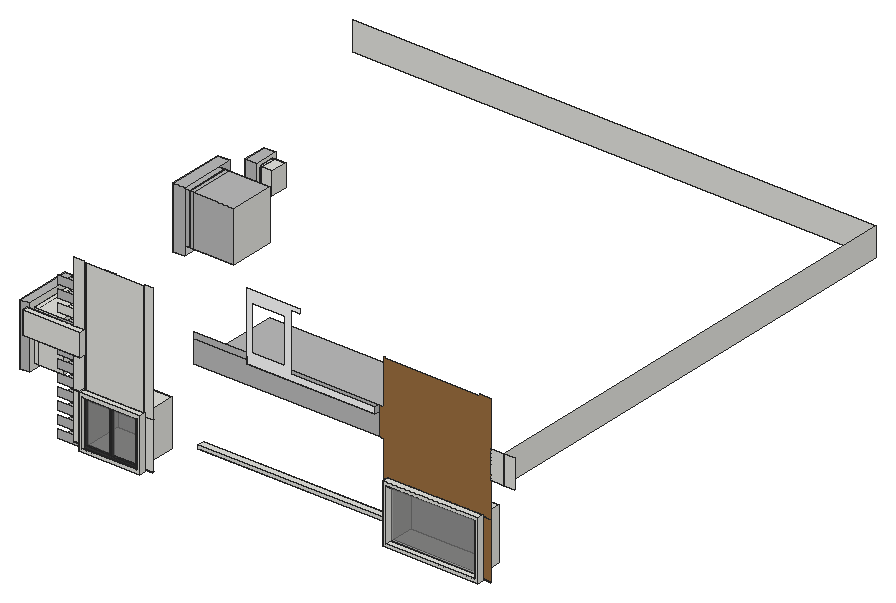
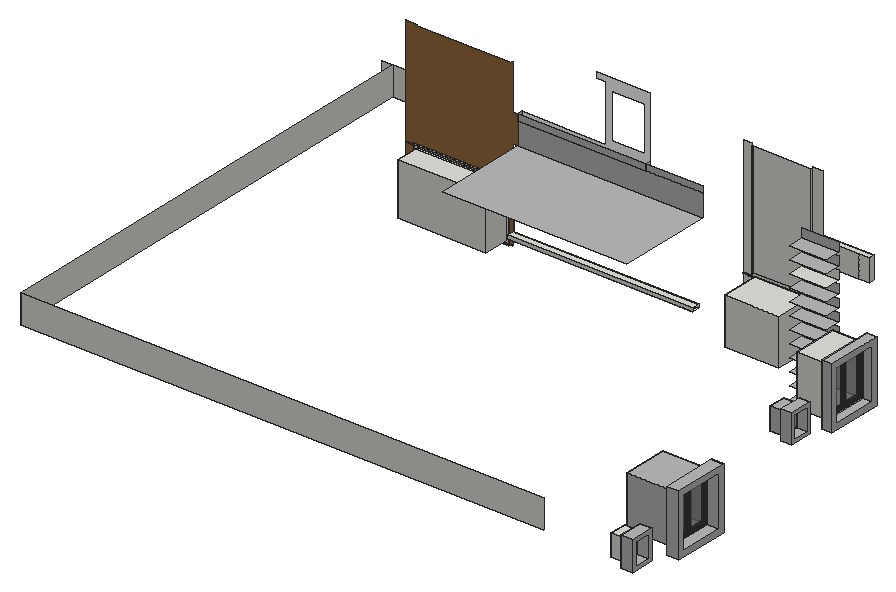
# SketchUp Ruby script. Lengths in inches.
U = 1.inch
M = Sketchup.active_model
def pt(a) = Geom::Point3d.new(a.map { |v| v * U })
def face(e, loops, mat)
  f = e.add_face(loops[0].map { |a| pt(a) })
  loops[1..].each { |l| e.add_face(l.map { |a| pt(a) }).erase! }
  f.material = f.back_material = mat if mat
  f
end
# faces: each face lists its corners as indices into pts; further lists are holes
def faces(e, pts, list, mat = nil) = list.each { |f| face(e, (f[0].is_a?(Array) ? f : [f]).map { |l| l.map { |i| pts[i] } }, mat) }
# xy, xz, yz: faces in a plane at the given z, y or x. An outline is a flat list of corners, or four numbers for a rectangle; further outlines are holes
def ring(l) = l.size == 4 ? [[l[0], l[1]], [l[2], l[1]], [l[2], l[3]], [l[0], l[3]]] : l.each_slice(2).to_a
def flat(e, list, mat, &to3) = list.each { |f| face(e, (f[0].is_a?(Array) ? f : [f]).map { |l| ring(l).map { |u, v| to3.(u, v) } }, mat) }
def xy(e, z, list, mat = nil) = flat(e, list, mat) { |x, y| [x, y, z] }
def xz(e, y, list, mat = nil) = flat(e, list, mat) { |x, z| [x, y, z] }
def yz(e, x, list, mat = nil) = flat(e, list, mat) { |y, z| [x, y, z] }
def lines(e, pts, list) = list.each { |a, b| e.add_line(pt(pts[a]), pt(pts[b])) }
# prism: a flat outline (further loops are holes) pulled along v
def prism(e, loops, v, mat = nil)
  f = face(e, loops, mat); d = Geom::Vector3d.new(v.map { |x| x * U })
  f.pushpull(f.normal.samedirection?(d) ? d.length : -d.length)
end
def box(e, o, s, mat = nil) = prism(e, [[o, [o[0] + s[0], o[1], o[2]], [o[0] + s[0], o[1] + s[1], o[2]], [o[0], o[1] + s[1], o[2]]]], [0, 0, s[2]], mat)
def at(x, y, z, deg = 0) = Geom::Transformation.translation(pt([x, y, z])) * Geom::Transformation.rotation(ORIGIN, Z_AXIS, deg.degrees)
def axes(o, x, y, z) = Geom::Transformation.new([*x, 0, *y, 0, *z, 0, *pt(o).to_a, 1])
def part(name) = M.definitions.add(name)
# library, detail: a bought-in or finely detailed component or shape, given as its bounding box
def library(name, o, s) = part(name).tap { |d| box(d.entities, o, s) }
def detail(e, o, s) = box(e.add_group.entities, o, s)
def put(e, d, t, mat = nil) = e.add_instance(d, t).tap { |i| i.material = mat if mat }
def group(e, t, mat = nil) = e.add_group.tap { |g| g.transformation = t; g.material = mat if mat }.entities
root = M.entities
M.materials.add("Generic").color = [155, 110, 63]
M.materials.add("Generic\#2").color = [186, 186, 186]
M.materials.add("[Color M00]").color = [255, 255, 255]
M.materials.add("[Color M07]").color = [58, 58, 58]
M.materials.add("[Translucent Glass Gray]").color = [127, 127, 127]
M.materials["[Translucent Glass Gray]"].alpha = 0.58
M.materials.add("[Translucent Glass Gray]1").color = [127, 127, 127]
M.materials["[Translucent Glass Gray]1"].alpha = 0.5
c1 = part("Group\#1")
xy(c1.entities,0,[[0,0,46.77,20.375]])
xz(c1.entities,0,[[0,0,46.77,11.0625]])
c2 = part("Group\#3")
xy(c2.entities,0,[[0,0,70.4375,6]],"[Color M07]")
xy(c2.entities,2.83,[[2.83,0,33.8,3],[36.63,0,67.61,3]],"[Color M07]")
xy(c2.entities,56.73,[[2.83,0,33.8,3],[36.63,0,67.61,3]],"[Color M07]")
xy(c2.entities,59.5625,[[0,0,70.4375,6]],"[Color M07]")
xz(c2.entities,0,[[[0,0,70.4375,59.5625],[2.83,2.83,33.8,56.73],[36.63,2.83,67.61,56.73]]],"[Color M07]")
xz(c2.entities,3,[[2.83,2.83,33.8,56.73],[36.63,2.83,67.61,56.73]],"[Translucent Glass Gray]")
xz(c2.entities,6,[[0,0,70.4375,59.5625]],"[Translucent Glass Gray]")
yz(c2.entities,0,[[0,0,6,59.5625]],"[Color M07]")
yz(c2.entities,2.83,[[0,2.83,3,56.73]],"[Color M07]")
yz(c2.entities,33.8,[[0,2.83,3,56.73]],"[Color M07]")
yz(c2.entities,36.63,[[0,2.83,3,56.73]],"[Color M07]")
yz(c2.entities,67.61,[[0,2.83,3,56.73]],"[Color M07]")
yz(c2.entities,70.4375,[[0,0,6,59.5625]],"[Color M07]")
c3 = part("Group\#2")
xy(c3.entities,0,[[0,0,113.875,3]])
xy(c3.entities,67.5625,[[0,0,113.875,3]])
xz(c3.entities,0,[[0,0,113.875,67.5625]],"[Translucent Glass Gray]")
xz(c3.entities,3,[[0,0,113.875,67.5625]],"[Translucent Glass Gray]")
yz(c3.entities,0,[[0,0,3,67.5625]])
yz(c3.entities,113.875,[[0,0,3,67.5625]])
c4 = part("Group\#4")
xy(c4.entities,0,[[0,0,6,57.4375]],"[Color M07]")
xy(c4.entities,5.48,[[0,5.48,3,25.98],[0,31.46,3,51.96]],"[Color M07]")
xy(c4.entities,59.46,[[0,5.48,3,25.98],[0,31.46,3,51.96]],"[Color M07]")
xy(c4.entities,64.9375,[[0,0,6,57.4375]],"[Color M07]")
xz(c4.entities,0,[[0,0,6,64.9375]],"[Color M07]")
xz(c4.entities,5.48,[[0,5.48,3,59.46]],"[Color M07]")
xz(c4.entities,25.98,[[0,5.48,3,59.46]],"[Color M07]")
xz(c4.entities,31.46,[[0,5.48,3,59.46]],"[Color M07]")
xz(c4.entities,51.96,[[0,5.48,3,59.46]],"[Color M07]")
xz(c4.entities,57.4375,[[0,0,6,64.9375]],"[Color M07]")
yz(c4.entities,0,[[[0,0,57.4375,64.9375],[31.46,5.48,51.96,59.46],[5.48,5.48,25.98,59.46]]],"[Color M07]")
yz(c4.entities,3,[[5.48,5.48,25.98,59.46],[31.46,5.48,51.96,59.46]],"[Translucent Glass Gray]1")
yz(c4.entities,6,[[0,0,57.4375,64.9375]],"[Translucent Glass Gray]1")
c5 = part("Group\#5")
xy(c5.entities,0,[[0,0,3,21.5625]])
xy(c5.entities,28.3125,[[0,0,3,21.5625]])
xz(c5.entities,0,[[0,0,3,28.3125]])
xz(c5.entities,21.5625,[[0,0,3,28.3125]])
yz(c5.entities,0,[[0,0,21.5625,28.3125]],"[Translucent Glass Gray]1")
yz(c5.entities,3,[[0,0,21.5625,28.3125]],"[Translucent Glass Gray]1")
xy(root,450.375,[[170.35,89.25,249.19,97.25],[171.66,97.25,172.16,98.375],[247.01,97.25,247.51,98.375]])
xy(root,453.4375,[[157.47,97.25,170.35,98.375],[249.19,97.25,259.3125,98.375]])
xy(root,453.9375,[[157.47,97.25,170.35,98.375],[249.19,97.25,259.3125,98.375]])
xy(root,454.58,[[174.55,89.25,244.99,97.25],[174.55,97.25,244.99,145.8125]])
xy(root,458.4,[[540.25,116.625,662.53,124.5]])
xy(root,461.15,[[0,454.08,15.3125,525.8]],"Generic\#2")
xy(root,462.6,[[544.45,116.625,658.33,124.5],[544.45,124.5,658.33,156.8125]])
xy(root,467.02,[[36.4375,161.95,48.5,234.18]],"Generic\#2")
xy(root,468.29,[[0,461.22,72.5625,518.66]],"Generic\#2")
xy(root,474.41,[[48.5,169.34,87,226.78]])
xy(root,474.41,[[36.4375,169.34,48.5,226.78]],"Generic\#2")
xy(root,477.08,[[[290.4375,131.37,528.75,140.67],[521.23,133.41,521.44,133.44,521.64,133.52,521.8,133.65,521.93,133.82,522.02,134.02,522.04,134.23,522.02,134.4375,521.93,134.63,521.8,134.8,521.64,134.93,521.44,135.01,521.23,135.04,521.02,135.01,520.82,134.93,520.66,134.8,520.53,134.63,520.45,134.4375,520.42,134.23,520.45,134.02,520.53,133.82,520.66,133.65,520.82,133.52,521.02,133.44],[515.92,133.41,516.13,133.44,516.32,133.52,516.49,133.65,516.62,133.82,516.7,134.02,516.73,134.23,516.7,134.4375,516.62,134.63,516.49,134.8,516.32,134.93,516.13,135.01,515.92,135.04,515.71,135.01,515.51,134.93,515.34,134.8,515.21,134.63,515.13,134.4375,515.11,134.23,515.13,134.02,515.21,133.82,515.34,133.65,515.51,133.52,515.71,133.44],[510.67,133.41,510.88,133.44,511.07,133.52,511.24,133.65,511.37,133.82,511.45,134.02,511.48,134.23,511.45,134.4375,511.37,134.63,511.24,134.8,511.07,134.93,510.88,135.01,510.67,135.04,510.46,135.01,510.26,134.93,510.09,134.8,509.96,134.63,509.88,134.4375,509.86,134.23,509.88,134.02,509.96,133.82,510.09,133.65,510.26,133.52,510.46,133.44],[505.42,133.41,505.63,133.44,505.82,133.52,505.99,133.65,506.12,133.82,506.2,134.02,506.23,134.23,506.2,134.4375,506.12,134.63,505.99,134.8,505.82,134.93,505.63,135.01,505.42,135.04,505.21,135.01,505.01,134.93,504.84,134.8,504.71,134.63,504.63,134.4375,504.61,134.23,504.63,134.02,504.71,133.82,504.84,133.65,505.01,133.52,505.21,133.44],[500.17,133.41,500.38,133.44,500.57,133.52,500.74,133.65,500.87,133.82,500.95,134.02,500.98,134.23,500.95,134.4375,500.87,134.63,500.74,134.8,500.57,134.93,500.38,135.01,500.17,135.04,499.96,135.01,499.76,134.93,499.59,134.8,499.46,134.63,499.38,134.4375,499.36,134.23,499.38,134.02,499.46,133.82,499.59,133.65,499.76,133.52,499.96,133.44],[494.86,133.41,495.07,133.44,495.26,133.52,495.43,133.65,495.56,133.82,495.64,134.02,495.67,134.23,495.64,134.4375,495.56,134.63,495.43,134.8,495.26,134.93,495.07,135.01,494.86,135.04,494.65,135.01,494.45,134.93,494.28,134.8,494.15,134.63,494.07,134.4375,494.04,134.23,494.07,134.02,494.15,133.82,494.28,133.65,494.45,133.52,494.65,133.44],[489.54,133.41,489.75,133.44,489.95,133.52,490.12,133.65,490.25,133.82,490.33,134.02,490.36,134.23,490.33,134.4375,490.25,134.63,490.12,134.8,489.95,134.93,489.75,135.01,489.54,135.04,489.33,135.01,489.14,134.93,488.97,134.8,488.84,134.63,488.76,134.4375,488.73,134.23,488.76,134.02,488.84,133.82,488.97,133.65,489.14,133.52,489.33,133.44],[483.92,133.41,484.13,133.44,484.32,133.52,484.49,133.65,484.62,133.82,484.7,134.02,484.73,134.23,484.7,134.4375,484.62,134.63,484.49,134.8,484.32,134.93,484.13,135.01,483.92,135.04,483.71,135.01,483.51,134.93,483.34,134.8,483.21,134.63,483.13,134.4375,483.11,134.23,483.13,134.02,483.21,133.82,483.34,133.65,483.51,133.52,483.71,133.44],[478.67,133.41,478.88,133.44,479.07,133.52,479.24,133.65,479.37,133.82,479.45,134.02,479.48,134.23,479.45,134.4375,479.37,134.63,479.24,134.8,479.07,134.93,478.88,135.01,478.67,135.04,478.46,135.01,478.26,134.93,478.09,134.8,477.96,134.63,477.88,134.4375,477.86,134.23,477.88,134.02,477.96,133.82,478.09,133.65,478.26,133.52,478.46,133.44],[473.42,133.41,473.63,133.44,473.82,133.52,473.99,133.65,474.12,133.82,474.2,134.02,474.23,134.23,474.2,134.4375,474.12,134.63,473.99,134.8,473.82,134.93,473.63,135.01,473.42,135.04,473.21,135.01,473.01,134.93,472.84,134.8,472.71,134.63,472.63,134.4375,472.61,134.23,472.63,134.02,472.71,133.82,472.84,133.65,473.01,133.52,473.21,133.44],[468.17,133.41,468.38,133.44,468.57,133.52,468.74,133.65,468.87,133.82,468.95,134.02,468.98,134.23,468.95,134.4375,468.87,134.63,468.74,134.8,468.57,134.93,468.38,135.01,468.17,135.04,467.96,135.01,467.76,134.93,467.59,134.8,467.46,134.63,467.38,134.4375,467.36,134.23,467.38,134.02,467.46,133.82,467.59,133.65,467.76,133.52,467.96,133.44],[462.92,133.41,463.13,133.44,463.32,133.52,463.49,133.65,463.62,133.82,463.7,134.02,463.73,134.23,463.7,134.4375,463.62,134.63,463.49,134.8,463.32,134.93,463.13,135.01,462.92,135.04,462.71,135.01,462.51,134.93,462.34,134.8,462.21,134.63,462.13,134.4375,462.11,134.23,462.13,134.02,462.21,133.82,462.34,133.65,462.51,133.52,462.71,133.44],[457.67,133.41,457.88,133.44,458.07,133.52,458.24,133.65,458.37,133.82,458.45,134.02,458.48,134.23,458.45,134.4375,458.37,134.63,458.24,134.8,458.07,134.93,457.88,135.01,457.67,135.04,457.46,135.01,457.26,134.93,457.09,134.8,456.96,134.63,456.88,134.4375,456.86,134.23,456.88,134.02,456.96,133.82,457.09,133.65,457.26,133.52,457.46,133.44],[452.36,133.41,452.57,133.44,452.76,133.52,452.93,133.65,453.06,133.82,453.14,134.02,453.17,134.23,453.14,134.4375,453.06,134.63,452.93,134.8,452.76,134.93,452.57,135.01,452.36,135.04,452.15,135.01,451.95,134.93,451.78,134.8,451.65,134.63,451.57,134.4375,451.54,134.23,451.57,134.02,451.65,133.82,451.78,133.65,451.95,133.52,452.15,133.44],[447.04,133.41,447.25,133.44,447.45,133.52,447.62,133.65,447.75,133.82,447.83,134.02,447.86,134.23,447.83,134.4375,447.75,134.63,447.62,134.8,447.45,134.93,447.25,135.01,447.04,135.04,446.83,135.01,446.64,134.93,446.47,134.8,446.34,134.63,446.26,134.4375,446.23,134.23,446.26,134.02,446.34,133.82,446.47,133.65,446.64,133.52,446.83,133.44],[441.73,133.41,441.94,133.44,442.14,133.52,442.3,133.65,442.43,133.82,442.52,134.02,442.54,134.23,442.52,134.4375,442.43,134.63,442.3,134.8,442.14,134.93,441.94,135.01,441.73,135.04,441.52,135.01,441.32,134.93,441.16,134.8,441.03,134.63,440.95,134.4375,440.92,134.23,440.95,134.02,441.03,133.82,441.16,133.65,441.32,133.52,441.52,133.44],[436.42,133.41,436.63,133.44,436.82,133.52,436.99,133.65,437.12,133.82,437.2,134.02,437.23,134.23,437.2,134.4375,437.12,134.63,436.99,134.8,436.82,134.93,436.63,135.01,436.42,135.04,436.21,135.01,436.01,134.93,435.84,134.8,435.71,134.63,435.63,134.4375,435.61,134.23,435.63,134.02,435.71,133.82,435.84,133.65,436.01,133.52,436.21,133.44],[431.11,133.41,431.32,133.44,431.51,133.52,431.68,133.65,431.81,133.82,431.89,134.02,431.92,134.23,431.89,134.4375,431.81,134.63,431.68,134.8,431.51,134.93,431.32,135.01,431.11,135.04,430.9,135.01,430.7,134.93,430.53,134.8,430.4,134.63,430.32,134.4375,430.29,134.23,430.32,134.02,430.4,133.82,430.53,133.65,430.7,133.52,430.9,133.44],[425.79,133.41,426,133.44,426.2,133.52,426.37,133.65,426.5,133.82,426.58,134.02,426.61,134.23,426.58,134.4375,426.5,134.63,426.37,134.8,426.2,134.93,426,135.01,425.79,135.04,425.58,135.01,425.39,134.93,425.22,134.8,425.09,134.63,425.01,134.4375,424.98,134.23,425.01,134.02,425.09,133.82,425.22,133.65,425.39,133.52,425.58,133.44],[420.48,133.41,420.69,133.44,420.89,133.52,421.05,133.65,421.18,133.82,421.27,134.02,421.29,134.23,421.27,134.4375,421.18,134.63,421.05,134.8,420.89,134.93,420.69,135.01,420.48,135.04,420.27,135.01,420.07,134.93,419.91,134.8,419.78,134.63,419.7,134.4375,419.67,134.23,419.7,134.02,419.78,133.82,419.91,133.65,420.07,133.52,420.27,133.44],[415.17,133.41,415.38,133.44,415.57,133.52,415.74,133.65,415.87,133.82,415.95,134.02,415.98,134.23,415.95,134.4375,415.87,134.63,415.74,134.8,415.57,134.93,415.38,135.01,415.17,135.04,414.96,135.01,414.76,134.93,414.59,134.8,414.46,134.63,414.38,134.4375,414.36,134.23,414.38,134.02,414.46,133.82,414.59,133.65,414.76,133.52,414.96,133.44],[409.86,133.41,410.07,133.44,410.26,133.52,410.43,133.65,410.56,133.82,410.64,134.02,410.67,134.23,410.64,134.4375,410.56,134.63,410.43,134.8,410.26,134.93,410.07,135.01,409.86,135.04,409.65,135.01,409.45,134.93,409.28,134.8,409.15,134.63,409.07,134.4375,409.04,134.23,409.07,134.02,409.15,133.82,409.28,133.65,409.45,133.52,409.65,133.44],[404.54,133.41,404.75,133.44,404.95,133.52,405.12,133.65,405.25,133.82,405.33,134.02,405.36,134.23,405.33,134.4375,405.25,134.63,405.12,134.8,404.95,134.93,404.75,135.01,404.54,135.04,404.33,135.01,404.14,134.93,403.97,134.8,403.84,134.63,403.76,134.4375,403.73,134.23,403.76,134.02,403.84,133.82,403.97,133.65,404.14,133.52,404.33,133.44],[399.23,133.41,399.44,133.44,399.64,133.52,399.8,133.65,399.93,133.82,400.02,134.02,400.04,134.23,400.02,134.4375,399.93,134.63,399.8,134.8,399.64,134.93,399.44,135.01,399.23,135.04,399.02,135.01,398.82,134.93,398.66,134.8,398.53,134.63,398.45,134.4375,398.42,134.23,398.45,134.02,398.53,133.82,398.66,133.65,398.82,133.52,399.02,133.44],[393.92,133.41,394.13,133.44,394.32,133.52,394.49,133.65,394.62,133.82,394.7,134.02,394.73,134.23,394.7,134.4375,394.62,134.63,394.49,134.8,394.32,134.93,394.13,135.01,393.92,135.04,393.71,135.01,393.51,134.93,393.34,134.8,393.21,134.63,393.13,134.4375,393.11,134.23,393.13,134.02,393.21,133.82,393.34,133.65,393.51,133.52,393.71,133.44],[388.61,133.41,388.82,133.44,389.01,133.52,389.18,133.65,389.31,133.82,389.39,134.02,389.42,134.23,389.39,134.4375,389.31,134.63,389.18,134.8,389.01,134.93,388.82,135.01,388.61,135.04,388.4,135.01,388.2,134.93,388.03,134.8,387.9,134.63,387.82,134.4375,387.79,134.23,387.82,134.02,387.9,133.82,388.03,133.65,388.2,133.52,388.4,133.44],[383.29,133.41,383.5,133.44,383.7,133.52,383.87,133.65,384,133.82,384.08,134.02,384.11,134.23,384.08,134.4375,384,134.63,383.87,134.8,383.7,134.93,383.5,135.01,383.29,135.04,383.08,135.01,382.89,134.93,382.72,134.8,382.59,134.63,382.51,134.4375,382.48,134.23,382.51,134.02,382.59,133.82,382.72,133.65,382.89,133.52,383.08,133.44],[377.98,133.41,378.19,133.44,378.39,133.52,378.55,133.65,378.68,133.82,378.77,134.02,378.79,134.23,378.77,134.4375,378.68,134.63,378.55,134.8,378.39,134.93,378.19,135.01,377.98,135.04,377.77,135.01,377.57,134.93,377.41,134.8,377.28,134.63,377.2,134.4375,377.17,134.23,377.2,134.02,377.28,133.82,377.41,133.65,377.57,133.52,377.77,133.44],[372.67,133.41,372.88,133.44,373.07,133.52,373.24,133.65,373.37,133.82,373.45,134.02,373.48,134.23,373.45,134.4375,373.37,134.63,373.24,134.8,373.07,134.93,372.88,135.01,372.67,135.04,372.46,135.01,372.26,134.93,372.09,134.8,371.96,134.63,371.88,134.4375,371.86,134.23,371.88,134.02,371.96,133.82,372.09,133.65,372.26,133.52,372.46,133.44],[367.36,133.41,367.57,133.44,367.76,133.52,367.93,133.65,368.06,133.82,368.14,134.02,368.17,134.23,368.14,134.4375,368.06,134.63,367.93,134.8,367.76,134.93,367.57,135.01,367.36,135.04,367.15,135.01,366.95,134.93,366.78,134.8,366.65,134.63,366.57,134.4375,366.54,134.23,366.57,134.02,366.65,133.82,366.78,133.65,366.95,133.52,367.15,133.44],[362.04,133.41,362.25,133.44,362.45,133.52,362.62,133.65,362.75,133.82,362.83,134.02,362.86,134.23,362.83,134.4375,362.75,134.63,362.62,134.8,362.45,134.93,362.25,135.01,362.04,135.04,361.83,135.01,361.64,134.93,361.47,134.8,361.34,134.63,361.26,134.4375,361.23,134.23,361.26,134.02,361.34,133.82,361.47,133.65,361.64,133.52,361.83,133.44],[356.73,133.41,356.94,133.44,357.14,133.52,357.3,133.65,357.43,133.82,357.52,134.02,357.54,134.23,357.52,134.4375,357.43,134.63,357.3,134.8,357.14,134.93,356.94,135.01,356.73,135.04,356.52,135.01,356.32,134.93,356.16,134.8,356.03,134.63,355.95,134.4375,355.92,134.23,355.95,134.02,356.03,133.82,356.16,133.65,356.32,133.52,356.52,133.44],[351.42,133.41,351.63,133.44,351.82,133.52,351.99,133.65,352.12,133.82,352.2,134.02,352.23,134.23,352.2,134.4375,352.12,134.63,351.99,134.8,351.82,134.93,351.63,135.01,351.42,135.04,351.21,135.01,351.01,134.93,350.84,134.8,350.71,134.63,350.63,134.4375,350.61,134.23,350.63,134.02,350.71,133.82,350.84,133.65,351.01,133.52,351.21,133.44],[346.11,133.41,346.32,133.44,346.51,133.52,346.68,133.65,346.81,133.82,346.89,134.02,346.92,134.23,346.89,134.4375,346.81,134.63,346.68,134.8,346.51,134.93,346.32,135.01,346.11,135.04,345.9,135.01,345.7,134.93,345.53,134.8,345.4,134.63,345.32,134.4375,345.29,134.23,345.32,134.02,345.4,133.82,345.53,133.65,345.7,133.52,345.9,133.44],[340.79,133.41,341,133.44,341.2,133.52,341.37,133.65,341.5,133.82,341.58,134.02,341.61,134.23,341.58,134.4375,341.5,134.63,341.37,134.8,341.2,134.93,341,135.01,340.79,135.04,340.58,135.01,340.39,134.93,340.22,134.8,340.09,134.63,340.01,134.4375,339.98,134.23,340.01,134.02,340.09,133.82,340.22,133.65,340.39,133.52,340.58,133.44],[335.48,133.41,335.69,133.44,335.89,133.52,336.05,133.65,336.18,133.82,336.27,134.02,336.29,134.23,336.27,134.4375,336.18,134.63,336.05,134.8,335.89,134.93,335.69,135.01,335.48,135.04,335.27,135.01,335.07,134.93,334.91,134.8,334.78,134.63,334.7,134.4375,334.67,134.23,334.7,134.02,334.78,133.82,334.91,133.65,335.07,133.52,335.27,133.44],[330.17,133.41,330.38,133.44,330.57,133.52,330.74,133.65,330.87,133.82,330.95,134.02,330.98,134.23,330.95,134.4375,330.87,134.63,330.74,134.8,330.57,134.93,330.38,135.01,330.17,135.04,329.96,135.01,329.76,134.93,329.59,134.8,329.46,134.63,329.38,134.4375,329.36,134.23,329.38,134.02,329.46,133.82,329.59,133.65,329.76,133.52,329.96,133.44],[324.86,133.41,325.07,133.44,325.26,133.52,325.43,133.65,325.56,133.82,325.64,134.02,325.67,134.23,325.64,134.4375,325.56,134.63,325.43,134.8,325.26,134.93,325.07,135.01,324.86,135.04,324.65,135.01,324.45,134.93,324.28,134.8,324.15,134.63,324.07,134.4375,324.04,134.23,324.07,134.02,324.15,133.82,324.28,133.65,324.45,133.52,324.65,133.44],[319.54,133.41,319.75,133.44,319.95,133.52,320.12,133.65,320.25,133.82,320.33,134.02,320.36,134.23,320.33,134.4375,320.25,134.63,320.12,134.8,319.95,134.93,319.75,135.01,319.54,135.04,319.33,135.01,319.14,134.93,318.97,134.8,318.84,134.63,318.76,134.4375,318.73,134.23,318.76,134.02,318.84,133.82,318.97,133.65,319.14,133.52,319.33,133.44],[314.23,133.41,314.44,133.44,314.64,133.52,314.8,133.65,314.93,133.82,315.02,134.02,315.04,134.23,315.02,134.4375,314.93,134.63,314.8,134.8,314.64,134.93,314.44,135.01,314.23,135.04,314.02,135.01,313.82,134.93,313.66,134.8,313.53,134.63,313.45,134.4375,313.42,134.23,313.45,134.02,313.53,133.82,313.66,133.65,313.82,133.52,314.02,133.44],[308.92,133.41,309.13,133.44,309.32,133.52,309.49,133.65,309.62,133.82,309.7,134.02,309.73,134.23,309.7,134.4375,309.62,134.63,309.49,134.8,309.32,134.93,309.13,135.01,308.92,135.04,308.71,135.01,308.51,134.93,308.34,134.8,308.21,134.63,308.13,134.4375,308.11,134.23,308.13,134.02,308.21,133.82,308.34,133.65,308.51,133.52,308.71,133.44],[303.61,133.41,303.82,133.44,304.01,133.52,304.18,133.65,304.31,133.82,304.39,134.02,304.42,134.23,304.39,134.4375,304.31,134.63,304.18,134.8,304.01,134.93,303.82,135.01,303.61,135.04,303.4,135.01,303.2,134.93,303.03,134.8,302.9,134.63,302.82,134.4375,302.79,134.23,302.82,134.02,302.9,133.82,303.03,133.65,303.2,133.52,303.4,133.44],[298.29,133.41,298.5,133.44,298.7,133.52,298.87,133.65,299,133.82,299.08,134.02,299.11,134.23,299.08,134.4375,299,134.63,298.87,134.8,298.7,134.93,298.5,135.01,298.29,135.04,298.08,135.01,297.89,134.93,297.72,134.8,297.59,134.63,297.51,134.4375,297.48,134.23,297.51,134.02,297.59,133.82,297.72,133.65,297.89,133.52,298.08,133.44],[292.92,133.41,293.13,133.44,293.32,133.52,293.49,133.65,293.62,133.82,293.7,134.02,293.73,134.23,293.7,134.4375,293.62,134.63,293.49,134.8,293.32,134.93,293.13,135.01,292.92,135.04,292.71,135.01,292.51,134.93,292.34,134.8,292.21,134.63,292.13,134.4375,292.11,134.23,292.13,134.02,292.21,133.82,292.34,133.65,292.51,133.52,292.71,133.44]]])
xy(root,478.92,[[0,569.42,15.3125,600.66]],"Generic\#2")
xy(root,481.27,[[290.4375,131.37,528.75,140.67]])
xy(root,482.8,[[34.5,270.92,48.5,300.91]],"Generic\#2")
xy(root,483.76,[[15.3125,574.26,31.25,595.82]])
xy(root,483.76,[[0,574.26,15.3125,595.82]],"Generic\#2")
xy(root,487.01,[[34.5,275.13,65.625,296.69]],"Generic\#2")
xy(root,512.07,[[15.3125,574.26,31.25,595.82]])
xy(root,512.07,[[0,574.26,15.3125,595.82]],"Generic\#2")
xy(root,513.6875,[[157.47,97.25,170.35,98.375],[249.19,97.25,259.3125,98.375]])
xy(root,514.14,[[174.55,89.25,244.99,97.25],[174.55,97.25,244.99,145.8125]])
xy(root,514.1875,[[157.47,97.25,170.35,98.375],[249.19,97.25,259.3125,98.375]])
xy(root,515.32,[[34.5,275.13,65.625,296.69]],"Generic\#2")
xy(root,516.91,[[0,569.42,15.3125,600.66]],"Generic\#2")
xy(root,518.34,[[170.35,89.25,249.19,97.25],[171.66,97.25,172.16,98.375],[247.01,97.25,247.51,98.375]])
xy(root,519.54,[[34.5,270.92,48.5,300.91]],"Generic\#2")
xy(root,530.16,[[544.45,116.625,658.33,124.5],[544.45,124.5,658.33,156.8125]])
xy(root,533.23,[[0,461.22,72.5625,518.66]],"Generic\#2")
xy(root,534.36,[[540.25,116.625,662.53,124.5]])
xy(root,539.35,[[48.5,169.34,87,226.78]])
xy(root,539.35,[[36.4375,169.34,48.5,226.78]],"Generic\#2")
xy(root,540.37,[[0,454.08,15.3125,525.8]],"Generic\#2")
xy(root,546.75,[[36.4375,161.95,48.5,234.18]],"Generic\#2")
xy(root,558.95,[[96.98,89.5625,171.66,97.25]])
xy(root,577.875,[[290.4375,124.5,528.75,246]],"Generic\#2")
xy(root,587.54,[[96.98,89.5625,171.66,97.25]])
xy(root,606.6875,[[363.4375,118.5625,528.75,124.5]],"Generic\#2")
xz(root,89.25,[[[170.35,450.375,249.19,518.34],[174.55,454.58,244.99,514.14]]])
xz(root,89.5625,[[96.98,558.95,171.66,587.54]])
xz(root,97.25,[[170.35,450.375,171.66,514.1875],[[171.66,450.375,247.01,514.1875],[174.55,454.58,244.99,514.14]],[247.01,450.375,249.19,514.1875],[157.47,453.9375,170.35,513.6875],[249.19,453.9375,259.3125,513.6875],
  [157.47,514.1875,170.35,514.1875,170.35,518.34,171.66,518.34,171.66,558.95,157.47,558.95],[170.35,514.1875,171.66,518.34],[171.66,514.1875,247.01,518.34],[247.01,514.1875,249.19,518.34],[249.19,514.1875,259.3125,514.1875,259.3125,667,249.19,667,249.19,664.625,247.51,664.625,247.51,518.34,249.19,518.34],
  [172.16,518.34,247.01,664.625],[96.98,558.95,110.7,587.54],[110.7,558.95,157.47,587.54],[157.47,558.95,171.66,587.54],[157.47,587.54,171.66,587.54,171.66,664.625,170.35,664.625,170.35,667,157.47,667]])
xz(root,98.375,[[157.47,453.4375,170.35,453.9375],[249.19,453.4375,259.3125,453.9375],[157.47,513.6875,170.35,514.1875],[249.19,513.6875,259.3125,514.1875],[171.66,518.34,172.16,664.625],
  [247.01,518.34,247.51,664.625]])
xz(root,116.625,[[[540.25,458.4,662.53,534.36],[544.45,462.6,658.33,530.16]]])
xz(root,118.5625,[[[363.4375,606.6875,528.75,606.6875,528.75,614.8125,419.5625,614.8125,419.5625,687.77,431.875,687.77,431.875,694.14,363.4375,694.14],[370.16,621.53,412.84,678.86]]],"[Color M00]")
xz(root,124.5,[[540.25,458.4,662.53,459.625],[540.25,459.625,662.53,460.125],[[540.25,460.125,662.53,532.25],[544.45,462.6,658.33,530.16]],[540.25,532.25,662.53,534.36],[673.48,577.875,690.4375,614.8125],
  [690.4375,577.875,703.6875,614.8125]])
xz(root,124.5,[[535.75,459.625,540.25,460.125],[662.53,459.625,673.48,460.125],[535.75,460.125,540.25,532.25],[662.53,460.125,673.48,531.75],[662.53,531.75,673.48,532.25],
  [535.75,532.25,540.25,532.25,540.25,534.36,662.53,534.36,662.53,532.25,673.48,532.25,673.48,672.25,658.53,672.25,658.53,670.65,536.25,670.65,536.25,672.25,535.75,672.25,535.75,614.8125,528.75,614.8125,528.75,577.875,535.75,577.875]],"Generic")
xz(root,124.5,[[290.4375,577.875,528.75,606.6875],[290.4375,606.6875,363.4375,614.8125],[363.4375,606.6875,528.75,614.8125]],"Generic\#2")
xz(root,131.37,[[290.4375,477.08,528.75,481.27]])
xz(root,140.67,[[290.4375,477.08,528.75,481.27]])
xz(root,145.8125,[[174.55,454.58,244.99,514.14]])
xz(root,156.8125,[[544.45,462.6,658.33,530.16]])
xz(root,161.95,[[36.4375,467.02,48.5,546.75]],"Generic\#2")
xz(root,169.34,[[48.5,474.41,87,539.35]])
xz(root,169.34,[[36.4375,474.41,48.5,539.35]],"Generic\#2")
xz(root,226.78,[[48.5,474.41,87,539.35]])
xz(root,226.78,[[36.4375,474.41,48.5,539.35]],"Generic\#2")
xz(root,234.18,[[36.4375,467.02,48.5,546.75]],"Generic\#2")
xz(root,270.92,[[34.5,482.8,48.5,519.54]],"Generic\#2")
xz(root,275.13,[[34.5,487.01,65.625,515.32]],"Generic\#2")
xz(root,296.69,[[34.5,487.01,65.625,515.32]],"Generic\#2")
xz(root,300.91,[[34.5,482.8,48.5,519.54]],"Generic\#2")
xz(root,454.08,[[0,461.15,15.3125,540.37]],"Generic\#2")
xz(root,461.22,[[0,468.29,72.5625,533.23]],"Generic\#2")
xz(root,518.66,[[0,468.29,72.5625,533.23]],"Generic\#2")
xz(root,525.8,[[0,461.15,15.3125,540.37]],"Generic\#2")
xz(root,569.42,[[0,478.92,15.3125,516.91]],"Generic\#2")
xz(root,574.26,[[15.3125,483.76,31.25,512.07]])
xz(root,574.26,[[0,483.76,15.3125,512.07]],"Generic\#2")
xz(root,595.82,[[15.3125,483.76,31.25,512.07]])
xz(root,595.82,[[0,483.76,15.3125,512.07]],"Generic\#2")
xz(root,600.66,[[0,478.92,15.3125,516.91]],"Generic\#2")
xz(root,724.5,[[15.3125,577.875,690.4375,614.8125]])
yz(root,0,[[[454.08,461.15,525.8,540.37],[461.22,468.29,518.66,533.23]],[[569.42,478.92,600.66,516.91],[574.26,483.76,595.82,512.07]]],"Generic\#2")
yz(root,15.3125,[[[569.42,478.92,600.66,516.91],[574.26,483.76,595.82,512.07]]])
yz(root,31.25,[[574.26,483.76,595.82,512.07]])
yz(root,34.5,[[[270.92,482.8,300.91,519.54],[275.13,487.01,296.69,515.32]]],"Generic\#2")
yz(root,36.4375,[[[161.95,467.02,234.18,546.75],[169.34,474.41,226.78,539.35]]],"Generic\#2")
yz(root,48.5,[[[161.95,467.02,234.18,546.75],[169.34,474.41,226.78,539.35]]])
yz(root,65.625,[[275.13,487.01,296.69,515.32]])
yz(root,72.5625,[[461.22,468.29,518.66,533.23]])
yz(root,87,[[169.34,474.41,226.78,539.35]])
yz(root,96.98,[[89.5625,558.95,97.25,587.54]])
yz(root,170.35,[[89.25,450.375,97.25,518.34],[97.25,453.4375,98.375,453.9375],[97.25,513.6875,98.375,514.1875]])
yz(root,171.66,[[97.25,518.34,98.375,558.95],[89.5625,558.95,97.25,587.54],[97.25,558.95,98.375,587.54],[97.25,587.54,98.375,664.625]])
yz(root,172.16,[[97.25,518.34,98.375,558.95],[97.25,558.95,98.375,587.54],[97.25,587.54,98.375,664.625]])
yz(root,174.55,[[89.25,454.58,97.25,514.14],[97.25,454.58,145.8125,514.14]])
yz(root,244.99,[[89.25,454.58,97.25,514.14],[97.25,454.58,145.8125,514.14]])
yz(root,247.01,[[97.25,518.34,98.375,558.95],[97.25,558.95,98.375,587.54],[97.25,587.54,98.375,664.625]])
yz(root,247.51,[[97.25,518.34,98.375,558.95],[97.25,558.95,98.375,587.54],[97.25,587.54,98.375,664.625]])
yz(root,249.19,[[89.25,450.375,97.25,518.34],[97.25,453.4375,98.375,453.9375],[97.25,513.6875,98.375,514.1875]])
yz(root,363.4375,[[118.5625,606.6875,124.5,614.8125]],"[Color M00]")
yz(root,528.75,[[118.5625,606.6875,124.5,614.8125]],"Generic\#2")
yz(root,540.25,[[116.625,458.4,124.5,534.36]])
yz(root,544.45,[[116.625,462.6,124.5,530.16],[124.5,462.6,156.8125,530.16]])
yz(root,658.33,[[116.625,462.6,124.5,530.16],[124.5,462.6,156.8125,530.16]])
yz(root,662.53,[[116.625,458.4,124.5,534.36]])
yz(root,690.4375,[[124.5,577.875,724.5,614.8125]])
p = [[528.75,136.34,478.77],[290.4375,136.34,478.77]]
lines(root,p,[[0,1]])
put(root,c1,at(110.7,130.3125,426.3125),"Generic\#2")
put(root,c1,at(110.7,130.3125,442.5),"Generic\#2")
put(root,c2,at(174.55,91.75,454.58))
put(root,c1,at(110.7,130.3125,458.6875),"Generic\#2")
put(root,c3,at(544.45,124.5,462.6))
put(root,c4,at(15.3125,461.22,468.29))
put(root,c4,at(48.5,169.34,474.41))
put(root,c1,at(110.7,130.3125,474.875),"Generic\#2")
put(root,c5,at(15.3125,574.26,483.76))
put(root,c5,at(48.5,275.13,487.01))
put(root,c1,at(110.7,130.3125,491.0625),"Generic\#2")
put(root,c1,at(110.7,130.3125,507.25),"Generic\#2")
put(root,c1,at(110.7,130.3125,523.4375),"Generic\#2")
put(root,c1,at(110.7,130.3125,539.625),"Generic\#2")
put(root,c1,at(110.7,130.3125,555.8125),"Generic\#2")
put(root,c1,at(110.7,130.3125,572))
put(root,c1,at(110.7,130.3125,588.1875),"Generic\#2")
put(root,c1,at(110.7,130.3125,604.375),"Generic\#2")
